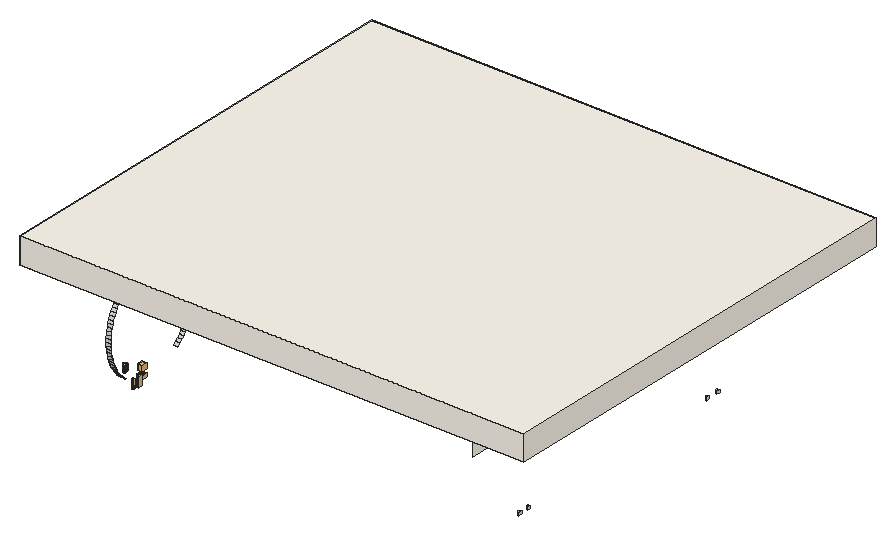
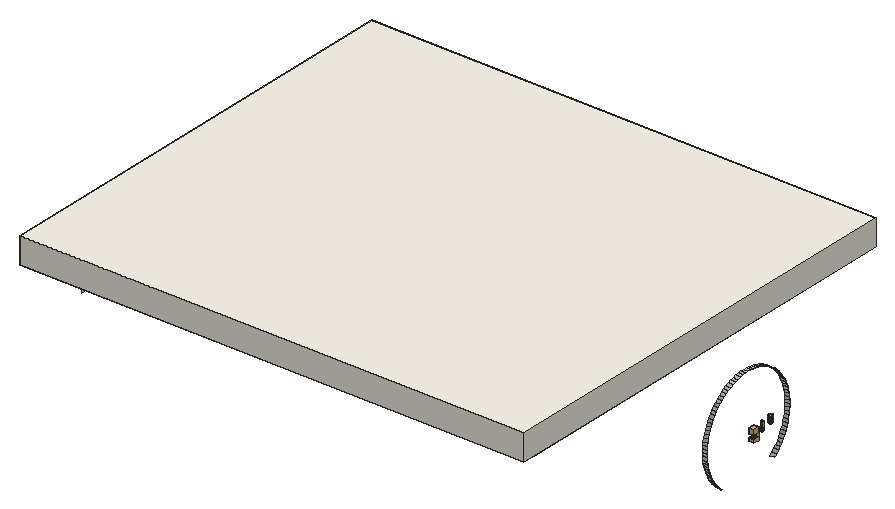
# SketchUp Ruby script. Lengths in inches.
U = 1.inch
M = Sketchup.active_model
def pt(a) = Geom::Point3d.new(a.map { |v| v * U })
def face(e, loops, mat)
  f = e.add_face(loops[0].map { |a| pt(a) })
  loops[1..].each { |l| e.add_face(l.map { |a| pt(a) }).erase! }
  f.material = f.back_material = mat if mat
  f
end
# faces: each face lists its corners as indices into pts; further lists are holes
def faces(e, pts, list, mat = nil) = list.each { |f| face(e, (f[0].is_a?(Array) ? f : [f]).map { |l| l.map { |i| pts[i] } }, mat) }
# xy, xz, yz: faces in a plane at the given z, y or x. An outline is a flat list of corners, or four numbers for a rectangle; further outlines are holes
def ring(l) = l.size == 4 ? [[l[0], l[1]], [l[2], l[1]], [l[2], l[3]], [l[0], l[3]]] : l.each_slice(2).to_a
def flat(e, list, mat, &to3) = list.each { |f| face(e, (f[0].is_a?(Array) ? f : [f]).map { |l| ring(l).map { |u, v| to3.(u, v) } }, mat) }
def xy(e, z, list, mat = nil) = flat(e, list, mat) { |x, y| [x, y, z] }
def xz(e, y, list, mat = nil) = flat(e, list, mat) { |x, z| [x, y, z] }
def yz(e, x, list, mat = nil) = flat(e, list, mat) { |y, z| [x, y, z] }
def lines(e, pts, list) = list.each { |a, b| e.add_line(pt(pts[a]), pt(pts[b])) }
# prism: a flat outline (further loops are holes) pulled along v
def prism(e, loops, v, mat = nil)
  f = face(e, loops, mat); d = Geom::Vector3d.new(v.map { |x| x * U })
  f.pushpull(f.normal.samedirection?(d) ? d.length : -d.length)
end
def box(e, o, s, mat = nil) = prism(e, [[o, [o[0] + s[0], o[1], o[2]], [o[0] + s[0], o[1] + s[1], o[2]], [o[0], o[1] + s[1], o[2]]]], [0, 0, s[2]], mat)
def at(x, y, z, deg = 0) = Geom::Transformation.translation(pt([x, y, z])) * Geom::Transformation.rotation(ORIGIN, Z_AXIS, deg.degrees)
def axes(o, x, y, z) = Geom::Transformation.new([*x, 0, *y, 0, *z, 0, *pt(o).to_a, 1])
def part(name) = M.definitions.add(name)
# library, detail: a bought-in or finely detailed component or shape, given as its bounding box
def library(name, o, s) = part(name).tap { |d| box(d.entities, o, s) }
def detail(e, o, s) = box(e.add_group.entities, o, s)
def put(e, d, t, mat = nil) = e.add_instance(d, t).tap { |i| i.material = mat if mat }
def group(e, t, mat = nil) = e.add_group.tap { |g| g.transformation = t; g.material = mat if mat }.entities
root = M.entities
M.materials.add("Tom-Ford-Neroli-Portofino-Edp-50ml-Erkek-Tester-Parfum-resim").color = [184, 200, 191]
M.materials.add("Versace-Pour-Homme-EDT-100ml-Erkek-Tester-Parfum-resim-2040").color = [225, 231, 235]
M.materials.add("[0052_FloralWhite]").color = [255, 250, 240]
M.materials.add("[0053_Ivory]").color = [255, 255, 240]
M.materials.add("[Color M08]").color = [30, 30, 30]
M.materials.add("[Mirror 02]").color = [216, 216, 216]
M.materials.add("lancome-miracle-bahar-kokusu-parfüm-çiçek-şeker-koku").color = [245, 229, 246]
xy(root,63.398,[[[18.166,42.644,18.281,42.66,18.389,42.708,18.481,42.784,18.552,42.883,18.596,42.999,18.611,43.123,18.596,43.247,18.552,43.363,18.481,43.462,18.389,43.538,18.281,43.586,18.166,43.602,18.051,43.586,17.943,43.538,17.851,43.462,17.78,43.363,17.736,43.247,17.721,43.123,17.736,42.999,17.78,42.883,17.851,42.784,17.943,42.708,18.051,42.66],[18.166,42.786,18.085,42.798,18.01,42.831,17.945,42.885,17.895,42.955,17.864,43.036,17.853,43.123,17.864,43.21,17.895,43.292,17.945,43.361,18.01,43.415,18.085,43.449,18.166,43.46,18.247,43.449,18.323,43.415,18.387,43.361,18.437,43.292,18.469,43.21,18.479,43.123,18.469,43.036,18.437,42.955,18.387,42.885,18.323,42.831,18.247,42.798]]],"lancome-miracle-bahar-kokusu-parfüm-çiçek-şeker-koku")
xy(root,67.763,[[13.726,42.705,13.493,42.77,13.284,42.897,13.113,43.079,12.991,43.302,12.927,43.551,12.925,43.81,12.986,44.06,13.104,44.285,13.273,44.469,13.48,44.6,13.712,44.669,13.952,44.671,14.185,44.606,14.394,44.478,14.565,44.297,14.687,44.074,14.751,43.825,14.752,43.566,14.692,43.316,14.573,43.091,14.405,42.907,14.198,42.776,13.966,42.707]])
xy(root,70.269,[[13.726,42.705,13.966,42.707,14.198,42.776,14.405,42.907,14.573,43.091,14.692,43.316,14.752,43.566,14.751,43.825,14.687,44.074,14.565,44.297,14.394,44.478,14.185,44.606,13.952,44.671,13.712,44.669,13.48,44.6,13.273,44.469,13.104,44.285,12.986,44.06,12.925,43.81,12.927,43.551,12.991,43.302,13.113,43.079,13.284,42.897,13.493,42.77]],"Versace-Pour-Homme-EDT-100ml-Erkek-Tester-Parfum-resim-2040")
xy(root,83.633,[[210,27.045,209.361,27.38,209.361,28.052,210,28.388],[210,32.232,209.361,32.568,209.361,33.239,210,33.575],[210,135.92,209.361,136.255,209.361,136.927,210,137.263],[210,141.92,209.361,142.255,209.361,142.927,210,143.263]])
xy(root,84.893,[[210,27.045,210,28.388,209.361,28.052,209.125,28.052,209.125,27.38,209.361,27.38],[210,32.232,210,33.575,209.361,33.239,209.125,33.239,209.125,32.568,209.361,32.568],[210,135.92,210,137.263,209.361,136.927,209.125,136.927,209.125,136.255,209.361,136.255],[210,141.92,210,143.263,209.361,142.927,209.125,142.927,209.125,142.255,209.361,142.255]])
xy(root,115.5,[[209,59.071,210,83.357],[209,84.857,210,110.643]],"[Color M08]")
xy(root,117,[[209,57.571,210,84.857],[209,84.857,210,112.143]],"[Color M08]")
xy(root,126,[[[6,0,6,198,36,198,36,197,37.44,197,37.44,198,38.88,198,38.88,197,40.32,197,40.32,198,41.76,198,41.76,197,43.2,197,43.2,198,44.64,198,44.64,197,46.08,197,46.08,198,47.52,198,47.52,197,48.96,197,48.96,198,50.4,198,50.4,197,51.84,197,51.84,198,53.28,198,53.28,197,54.72,197,54.72,198,56.16,198,56.16,197,57.6,197,57.6,198,59.04,198,59.04,197,60.48,197,60.48,198,61.92,198,61.92,197,63.36,197,63.36,198,64.8,198,64.8,197,66.24,197,66.24,198,67.68,198,67.68,197,69.12,197,69.12,198,70.56,198,70.56,197,72,197,72,198,168,198,168,197,169.44,197,169.44,198,170.88,198,170.88,197,172.32,197,172.32,198,173.76,198,173.76,197,175.2,197,175.2,198,176.64,198,176.64,197,178.08,197,178.08,198,179.52,198,179.52,197,180.96,197,180.96,198,182.4,198,182.4,197,183.84,197,183.84,198,185.28,198,185.28,197,186.72,197,186.72,198,188.16,198,188.16,197,189.6,197,189.6,198,191.04,198,191.04,197,192.48,197,192.48,198,193.92,198,193.92,197,195.36,197,195.36,198,196.8,198,196.8,197,198.24,197,198.24,198,199.68,198,199.68,197,201.12,197,201.12,198,202.56,198,202.56,197,204,197,204,198,210,198,210,0],[30,24,186,174]]],"[0052_FloralWhite]")
xy(root,126,[[0,0,6,198],[210,0,234,198],[36,197,36,198,0,198,0,204,234,204,234,198,204,198,204,197,202.56,197,202.56,198,201.12,198,201.12,197,199.68,197,199.68,198,198.24,198,198.24,197,196.8,197,196.8,198,195.36,198,195.36,197,193.92,197,193.92,198,192.48,198,192.48,197,191.04,197,191.04,198,189.6,198,189.6,197,188.16,197,188.16,198,186.72,198,186.72,197,185.28,197,185.28,198,183.84,198,183.84,197,182.4,197,182.4,198,180.96,198,180.96,197,179.52,197,179.52,198,178.08,198,178.08,197,176.64,197,176.64,198,175.2,198,175.2,197,173.76,197,173.76,198,172.32,198,172.32,197,170.88,197,170.88,198,169.44,198,169.44,197,168,197,168,198,72,198,72,197,70.56,197,70.56,198,69.12,198,69.12,197,67.68,197,67.68,198,66.24,198,66.24,197,64.8,197,64.8,198,63.36,198,63.36,197,61.92,197,61.92,198,60.48,198,60.48,197,59.04,197,59.04,198,57.6,198,57.6,197,56.16,197,56.16,198,54.72,198,54.72,197,53.28,197,53.28,198,51.84,198,51.84,197,50.4,197,50.4,198,48.96,198,48.96,197,47.52,197,47.52,198,46.08,198,46.08,197,44.64,197,44.64,198,43.2,198,43.2,197,41.76,197,41.76,198,40.32,198,40.32,197,38.88,197,38.88,198,37.44,198,37.44,197]],"[0053_Ivory]")
xy(root,130,[[30,24,186,174]],"[0052_FloralWhite]")
xy(root,138,[[0,0,234,204]],"[0052_FloralWhite]")
xz(root,0,[[0,126,234,138]],"[0052_FloralWhite]")
xz(root,24,[[30,126,186,130]],"[0052_FloralWhite]")
xz(root,174,[[30,126,186,130]],"[0052_FloralWhite]")
xz(root,204,[[0,126,234,138]],"[0052_FloralWhite]")
yz(root,0,[[0,126,204,138]],"[0052_FloralWhite]")
yz(root,30,[[24,126,174,130]],"[0052_FloralWhite]")
yz(root,186,[[24,126,174,130]],"[0052_FloralWhite]")
yz(root,210,[[27.045,83.633,28.388,84.893],[32.232,83.633,33.575,84.893],[135.92,83.633,137.263,84.893],[141.92,83.633,143.263,84.893]])
yz(root,210,[[0,120,198,126]],"[0052_FloralWhite]")
yz(root,234,[[0,126,204,138]],"[0052_FloralWhite]")
p = [[6,50.115,59.831],[6,51.246,58.833],[8,51.246,58.833],[8,50.115,59.831],[6,81.843,58.833],[6,82.974,59.831],
  [8,82.974,59.831],[8,81.843,58.833],[6,49.049,60.897],[8,49.049,60.897],[6,84.04,60.897],[8,84.04,60.897],
  [6,48.052,62.028],[8,48.052,62.028],[6,85.037,62.028],[8,85.037,62.028],[18.166,42.644,62.012],[18.166,42.644,63.398],
  [18.051,42.66,63.398],[18.051,42.66,62.012],[18.281,42.66,62.012],[18.281,42.66,63.398],[17.943,42.708,62.012],[17.943,42.708,63.398],
  [17.851,42.784,63.398],[17.851,42.784,62.012],[18.389,42.708,62.012],[18.389,42.708,63.398],[18.481,42.784,62.012],[18.481,42.784,63.398],
  [17.78,42.883,63.398],[17.78,42.883,62.012],[18.552,42.883,62.012],[18.552,42.883,63.398],[17.736,42.999,63.398],[17.736,42.999,62.012],
  [18.596,42.999,62.012],[18.596,42.999,63.398],[17.721,43.123,63.398],[17.721,43.123,62.012],[18.611,43.123,62.012],[18.611,43.123,63.398],
  [17.736,43.247,63.398],[17.736,43.247,62.012],[18.596,43.247,62.012],[18.596,43.247,63.398],[17.78,43.363,63.398],[17.78,43.363,62.012],
  [18.552,43.363,62.012],[18.552,43.363,63.398],[17.851,43.462,63.398],[17.851,43.462,62.012],[18.481,43.462,62.012],[18.481,43.462,63.398],
  [17.943,43.538,63.398],[17.943,43.538,62.012],[18.051,43.586,63.398],[18.051,43.586,62.012],[18.281,43.586,62.012],[18.281,43.586,63.398],
  [18.389,43.538,63.398],[18.389,43.538,62.012],[18.166,43.602,63.398],[18.166,43.602,62.012],[6,47.128,63.219],[8,47.128,63.219],
  [6,85.961,63.219],[8,85.961,63.219],[6,46.281,64.466],[8,46.281,64.466],[6,86.808,64.466],[8,86.808,64.466],
  [15.548,50.496,65.573],[15.383,50.57,65.573],[15.383,50.57,63.593],[15.548,50.496,63.593],[15.725,50.471,65.573],[15.725,50.471,63.593],
  [15.902,50.496,65.573],[15.902,50.496,63.593],[16.067,50.57,65.573],[16.067,50.57,63.593],[15.241,50.687,65.573],[15.241,50.687,63.593],
  [16.208,50.687,65.573],[16.208,50.687,63.593],[15.133,50.839,65.573],[15.133,50.839,63.593],[16.317,50.839,65.573],[16.317,50.839,63.593],
  [15.064,51.016,65.573],[15.064,51.016,63.593],[16.385,51.016,65.573],[16.385,51.016,63.593],[15.041,51.207,65.573],[15.041,51.207,63.593],
  [16.408,51.207,65.573],[16.408,51.207,63.593],[15.064,51.397,65.573],[15.064,51.397,63.593],[16.385,51.397,65.573],[16.385,51.397,63.593],
  [15.133,51.575,65.573],[15.133,51.575,63.593],[16.317,51.575,65.573],[16.317,51.575,63.593],[15.241,51.727,65.573],[15.241,51.727,63.593],
  [16.208,51.727,65.573],[16.208,51.727,63.593],[15.383,51.844,65.573],[15.383,51.844,63.593],[16.067,51.844,65.573],[16.067,51.844,63.593],
  [15.548,51.918,65.573],[15.548,51.918,63.593],[15.902,51.918,65.573],[15.902,51.918,63.593],[15.725,51.943,65.573],[15.725,51.943,63.593],
  [6,45.513,65.764],[8,45.513,65.764],[6,87.576,65.764],[8,87.576,65.764],[6,44.829,67.107],[8,44.829,67.107],
  [6,88.26,67.107],[8,88.26,67.107],[13.764,43.04,67.739],[13.61,43.083,67.739],[13.61,43.083,67.137],[13.764,43.04,67.137],
  [13.923,43.041,67.739],[13.923,43.041,67.137],[14.076,43.086,67.739],[14.076,43.086,67.137],[13.472,43.167,67.739],[13.472,43.167,67.137],
  [14.213,43.173,67.739],[14.213,43.173,67.137],[13.359,43.287,67.739],[13.359,43.287,67.137],[14.324,43.295,67.739],[14.324,43.295,67.137],
  [13.278,43.434,67.739],[13.278,43.434,67.137],[14.403,43.443,67.739],[14.403,43.443,67.137],[13.236,43.599,67.739],[13.236,43.599,67.137],
  [14.442,43.609,67.739],[14.442,43.609,67.137],[13.235,43.77,67.739],[13.235,43.77,67.137],[14.441,43.78,67.739],[14.441,43.78,67.137],
  [13.275,43.935,67.739],[13.275,43.935,67.137],[14.399,43.945,67.739],[14.399,43.945,67.137],[13.353,44.084,67.739],[13.353,44.084,67.137],
  [14.319,44.092,67.739],[14.319,44.092,67.137],[13.465,44.206,67.739],[13.465,44.206,67.137],[14.205,44.212,67.739],[14.205,44.212,67.137],
  [6,44.23,68.491],[8,44.23,68.491],[13.602,44.292,67.739],[13.602,44.292,67.137],[14.067,44.296,67.739],[14.067,44.296,67.137],
  [13.755,44.338,67.739],[13.755,44.338,67.137],[13.913,44.339,67.739],[13.913,44.339,67.137],[6,88.859,68.491],[8,88.859,68.491],
  [13.726,42.705,70.269],[13.493,42.77,70.269],[13.493,42.77,67.763],[13.726,42.705,67.763],[13.966,42.707,70.269],[13.966,42.707,67.763],
  [14.198,42.776,70.269],[14.198,42.776,67.763],[13.284,42.897,70.269],[13.284,42.897,67.763],[14.405,42.907,70.269],[14.405,42.907,67.763],
  [13.113,43.079,70.269],[13.113,43.079,67.763],[14.573,43.091,70.269],[14.573,43.091,67.763],[12.991,43.302,70.269],[12.991,43.302,67.763],
  [14.692,43.316,70.269],[14.692,43.316,67.763],[12.927,43.551,70.269],[12.927,43.551,67.763],[14.752,43.566,70.269],[14.752,43.566,67.763],
  [12.925,43.81,70.269],[12.925,43.81,67.763],[14.751,43.825,70.269],[14.751,43.825,67.763],[12.986,44.06,70.269],[12.986,44.06,67.763],
  [14.687,44.074,70.269],[14.687,44.074,67.763],[13.104,44.285,70.269],[13.104,44.285,67.763],[14.565,44.297,70.269],[14.565,44.297,67.763],
  [13.273,44.469,70.269],[13.273,44.469,67.763],[14.394,44.478,70.269],[14.394,44.478,67.763],[13.48,44.6,70.269],[13.48,44.6,67.763],
  [14.185,44.606,70.269],[14.185,44.606,67.763],[13.712,44.669,70.269],[13.712,44.669,67.763],[13.952,44.671,70.269],[13.952,44.671,67.763],
  [6,43.719,69.909],[8,43.719,69.909],[6,89.37,69.909],[8,89.37,69.909],[6,43.299,71.357],[8,43.299,71.357],
  [6,89.791,71.357],[8,89.791,71.357],[6,42.97,72.829],[8,42.97,72.829],[6,90.119,72.829],[8,90.119,72.829],
  [6,42.734,74.318],[8,42.734,74.318],[6,90.355,74.318],[8,90.355,74.318],[6,42.592,75.819],[8,42.592,75.819],
  [6,90.497,75.819],[8,90.497,75.819],[6,42.545,77.326],[8,42.545,77.326],[6,90.545,77.326],[8,90.545,77.326],
  [6,42.592,78.833],[8,42.592,78.833],[6,90.497,78.833],[8,90.497,78.833],[6,42.734,80.334],[8,42.734,80.334],
  [6,90.355,80.334],[8,90.355,80.334],[6,42.97,81.823],[8,42.97,81.823],[6,90.119,81.823],[8,90.119,81.823],
  [6,43.299,83.294],[8,43.299,83.294],[6,89.791,83.294],[8,89.791,83.294],[6,43.719,84.742],[8,43.719,84.742],
  [6,89.37,84.742],[8,89.37,84.742],[210,27.045,84.893],[209.361,27.38,84.893],[209.361,27.38,83.633],[210,27.045,83.633],
  [209.361,28.052,84.893],[210,28.388,84.893],[210,28.388,83.633],[209.361,28.052,83.633],[210,32.232,84.893],[209.361,32.568,84.893],
  [209.361,32.568,83.633],[210,32.232,83.633],[209.361,33.239,84.893],[210,33.575,84.893],[210,33.575,83.633],[209.361,33.239,83.633],
  [210,135.92,84.893],[209.361,136.255,84.893],[209.361,136.255,83.633],[210,135.92,83.633],[209.361,136.927,84.893],[210,137.263,84.893],
  [210,137.263,83.633],[209.361,136.927,83.633],[210,141.92,84.893],[209.361,142.255,84.893],[209.361,142.255,83.633],[210,141.92,83.633],
  [209.361,142.927,84.893],[210,143.263,84.893],[210,143.263,83.633],[209.361,142.927,83.633],[6,44.23,86.161],[8,44.23,86.161],
  [6,88.859,86.161],[8,88.859,86.161],[6,44.829,87.545],[8,44.829,87.545],[6,88.26,87.545],[8,88.26,87.545],
  [6,45.513,88.888],[8,45.513,88.888],[6,87.576,88.888],[8,87.576,88.888],[6,46.281,90.186],[8,46.281,90.186],
  [6,86.808,90.186],[8,86.808,90.186],[6,47.128,91.433],[8,47.128,91.433],[6,85.961,91.433],[8,85.961,91.433],
  [6,48.052,92.624],[8,48.052,92.624],[6,85.037,92.624],[8,85.037,92.624],[6,49.049,93.755],[8,49.049,93.755],
  [6,84.04,93.755],[8,84.04,93.755],[6,50.115,94.821],[8,50.115,94.821],[6,82.974,94.821],[8,82.974,94.821],
  [6,51.246,95.818],[8,51.246,95.818],[6,81.843,95.818],[8,81.843,95.818],[6,52.4375,96.742],[8,52.4375,96.742],
  [6,80.651,96.742],[8,80.651,96.742],[6,53.685,97.59],[8,53.685,97.59],[6,79.404,97.59],[8,79.404,97.59],
  [6,54.982,98.357],[8,54.982,98.357],[6,78.107,98.357],[8,78.107,98.357],[6,56.326,99.042],[8,56.326,99.042],
  [6,76.763,99.042],[8,76.763,99.042],[6,57.71,99.64],[8,57.71,99.64],[6,75.38,99.64],[8,75.38,99.64],
  [6,59.128,100.151],[8,59.128,100.151],[6,73.961,100.151],[8,73.961,100.151],[6,60.576,100.572],[8,60.576,100.572],
  [6,72.513,100.572],[8,72.513,100.572],[6,62.047,100.901],[8,62.047,100.901],[6,71.042,100.901],[8,71.042,100.901],
  [6,63.537,101.137],[8,63.537,101.137],[6,69.553,101.137],[8,69.553,101.137],[6,65.038,101.278],[8,65.038,101.278],
  [6,68.052,101.278],[8,68.052,101.278],[6,66.545,101.326],[8,66.545,101.326],[16.811,49.945,66.613],[16.811,49.945,66.605],
  [12.896,47.663,69.872],[12.892,47.671,69.872]]
faces(root,p,[[0,1,2,3],[4,5,6,7],[8,0,3,9],[5,10,11,6],[12,8,9,13],[10,14,15,11],[64,12,13,65],[14,66,67,15],
  [68,64,65,69],[66,70,71,67],[120,68,69,121],[70,122,123,71],[124,120,121,125],[122,126,127,123],[168,124,125,169],[126,178,179,127],
  [228,168,169,229],[178,230,231,179],[232,228,229,233],[230,234,235,231],[236,232,233,237],[234,238,239,235],[240,236,237,241],[238,242,243,239],
  [244,240,241,245],[242,246,247,243],[248,244,245,249],[246,250,251,247],[252,248,249,253],[250,254,255,251],[256,252,253,257],[254,258,259,255],
  [260,256,257,261],[258,262,263,259],[264,260,261,265],[262,266,267,263],[268,264,265,269],[266,270,271,267],[304,268,269,305],[270,306,307,271],
  [308,304,305,309],[306,310,311,307],[312,308,309,313],[310,314,315,311],[316,312,313,317],[314,318,319,315],[320,316,317,321],[318,322,323,319],
  [324,320,321,325],[322,326,327,323],[328,324,325,329],[326,330,331,327],[332,328,329,333],[330,334,335,331],[336,332,333,337],[334,338,339,335],
  [340,336,337,341],[338,342,343,339],[344,340,341,345],[342,346,347,343],[348,344,345,349],[346,350,351,347],[352,348,349,353],[350,354,355,351],
  [356,352,353,357],[354,358,359,355],[360,356,357,361],[358,362,363,359],[364,360,361,365],[362,366,367,363],[368,364,365,369],[366,370,371,367],
  [372,368,369,373],[370,374,375,371],[376,372,373,377],[374,378,379,375],[380,376,377,381],[378,380,381,379]],"[Mirror 02]")
faces(root,p,[[16,17,18,19],[20,21,17,16],[22,23,24,25],[19,18,23,22],[26,27,21,20],[28,29,27,26],[25,24,30,31],[32,33,29,28],
  [31,30,34,35],[36,37,33,32],[35,34,38,39],[40,41,37,36],[39,38,42,43],[44,45,41,40],[43,42,46,47],[48,49,45,44],
  [47,46,50,51],[52,53,49,48],[51,50,54,55],[55,54,56,57],[58,59,60,61],[61,60,53,52],[57,56,62,63],[63,62,59,58]],"lancome-miracle-bahar-kokusu-parfüm-çiçek-şeker-koku")
faces(root,p,[[72,73,74,75],[76,72,75,77],[78,76,77,79],[80,78,79,81],[73,82,83,74],[84,80,81,85],[82,86,87,83],[88,84,85,89],
  [86,90,91,87],[92,88,89,93],[90,94,95,91],[96,92,93,97],[94,98,99,95],[100,96,97,101],[98,102,103,99],[104,100,101,105],
  [102,106,107,103],[108,104,105,109],[106,110,111,107],[112,108,109,113],[110,114,115,111],[116,112,113,117],[114,118,119,115],[118,116,117,119]],"Tom-Ford-Neroli-Portofino-Edp-50ml-Erkek-Tester-Parfum-resim")
faces(root,p,[[128,129,130,131],[132,128,131,133],[134,132,133,135],[129,136,137,130],[138,134,135,139],[136,140,141,137],[142,138,139,143],[140,144,145,141],
  [146,142,143,147],[144,148,149,145],[150,146,147,151],[148,152,153,149],[154,150,151,155],[152,156,157,153],[158,154,155,159],[156,160,161,157],
  [162,158,159,163],[160,164,165,161],[166,162,163,167],[164,170,171,165],[172,166,167,173],[170,174,175,171],[174,176,177,175],[176,172,173,177],
  [180,181,182,183],[184,180,183,185],[186,184,185,187],[181,188,189,182],[190,186,187,191],[188,192,193,189],[194,190,191,195],[192,196,197,193],
  [198,194,195,199],[196,200,201,197],[202,198,199,203],[200,204,205,201],[206,202,203,207],[204,208,209,205],[210,206,207,211],[208,212,213,209],
  [214,210,211,215],[212,216,217,213],[218,214,215,219],[216,220,221,217],[222,218,219,223],[220,224,225,221],[226,222,223,227],[224,226,227,225]],"Versace-Pour-Homme-EDT-100ml-Erkek-Tester-Parfum-resim-2040")
faces(root,p,[[272,273,274,275],[276,277,278,279],[280,281,282,283],[284,285,286,287],[288,289,290,291],[292,293,294,295],[296,297,298,299],[300,301,302,303]])
lines(root,p,[[382,383],[384,385]])
detail(root,[16.9,46.45,60.92],[1.31,1.42,4.62])
detail(root,[14.56,49.9375,62.26],[2.39,2.54,1.49])
detail(root,[17.72,42.6,63.41],[0.93,1.01,2.71])
detail(root,[14.61,49.91,65.54],[2.2,2.66,2.37])
